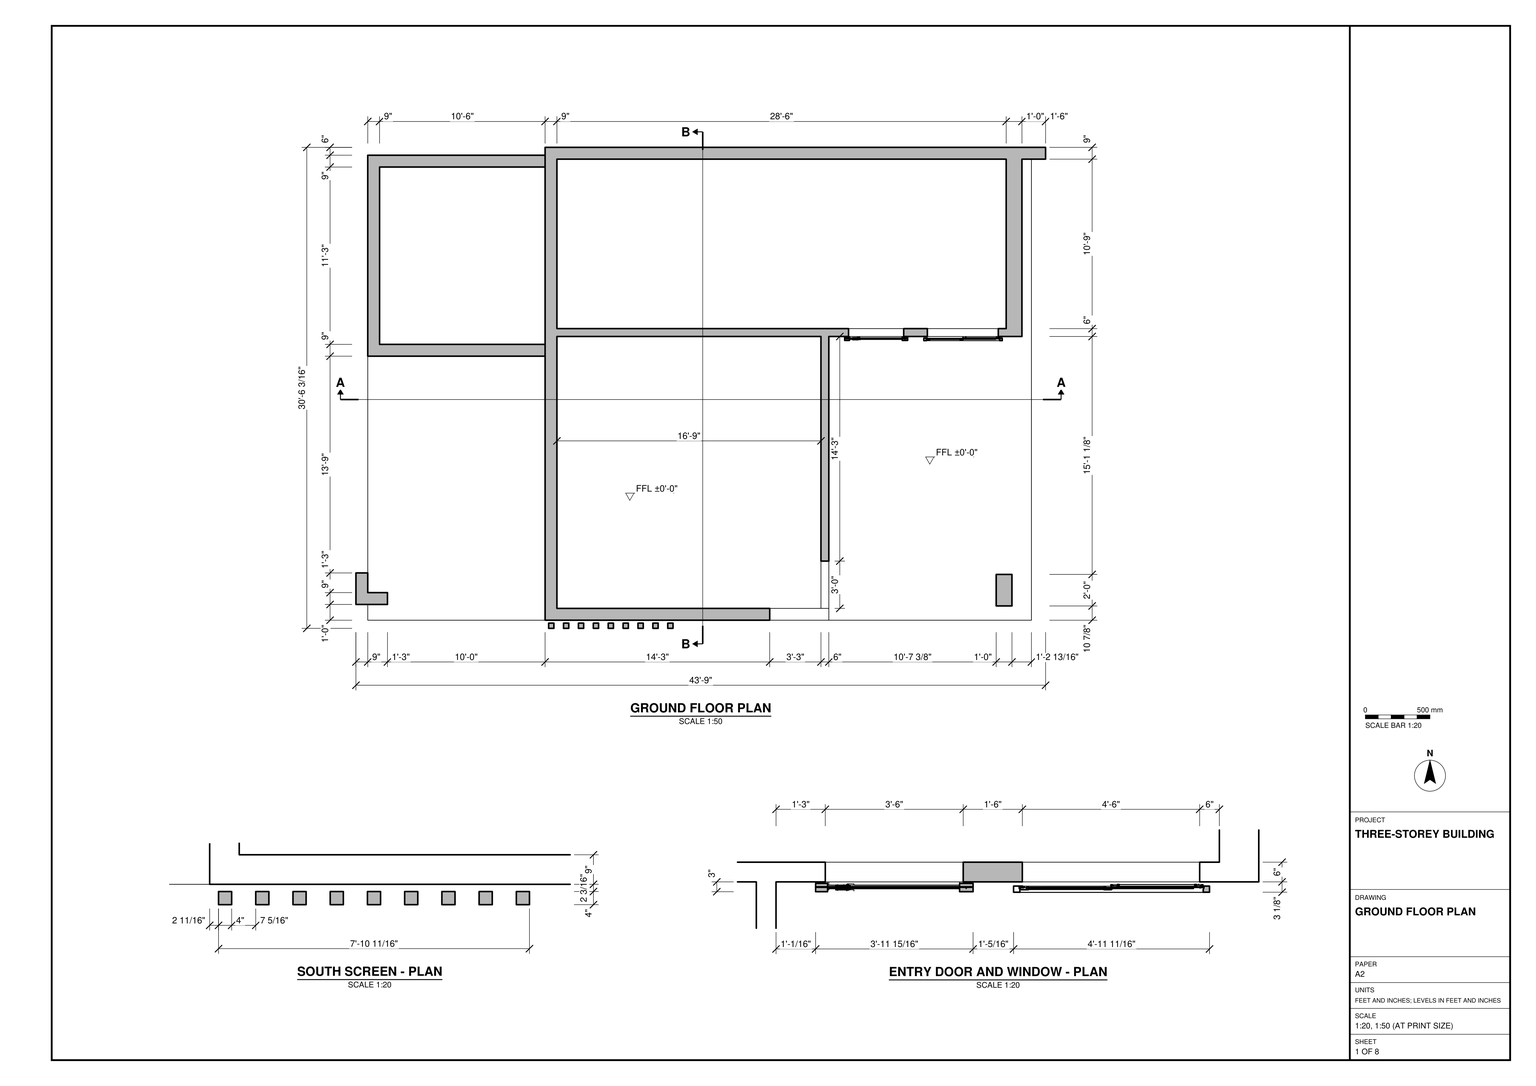
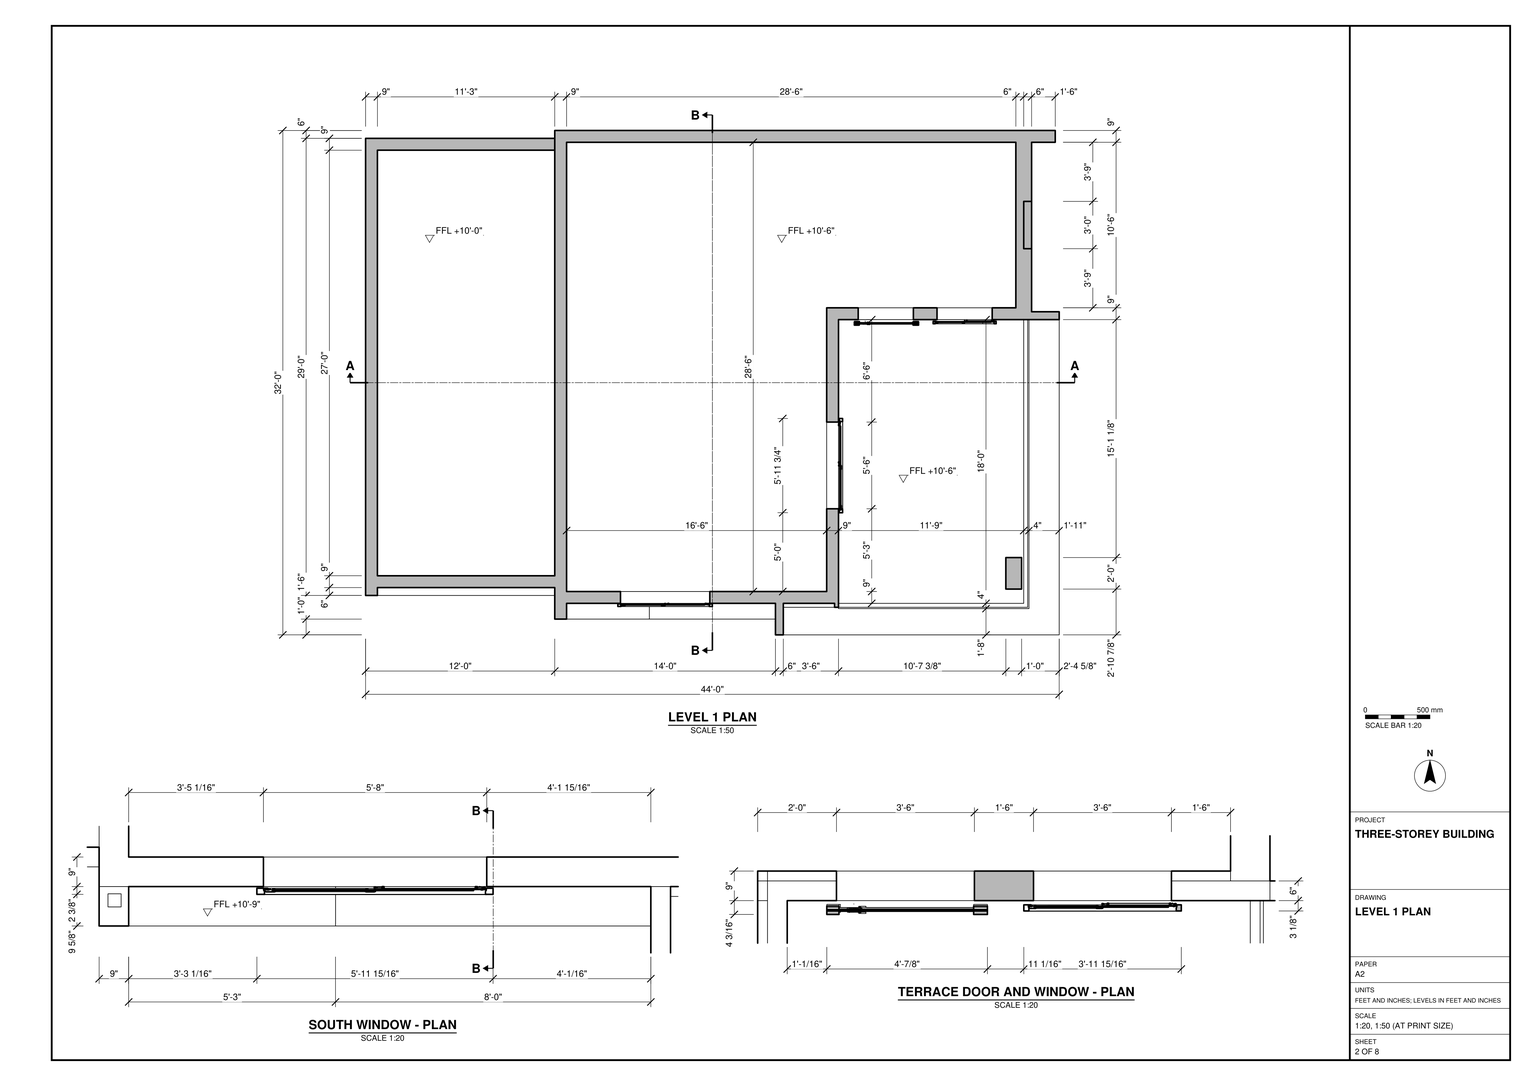
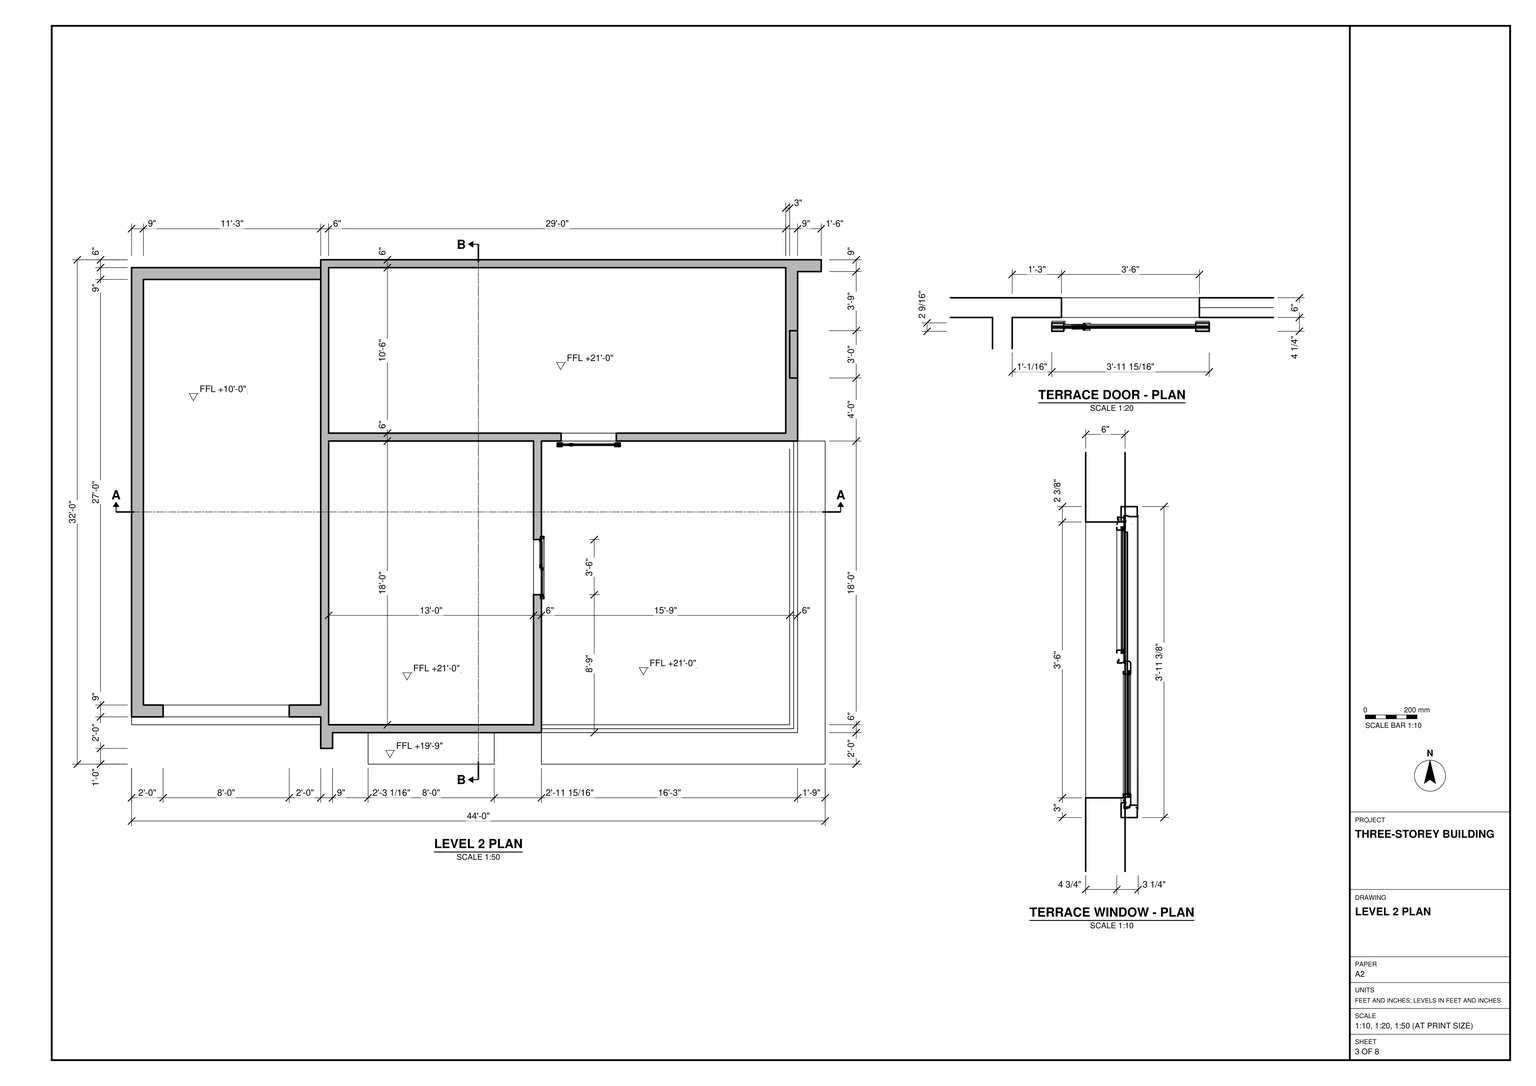
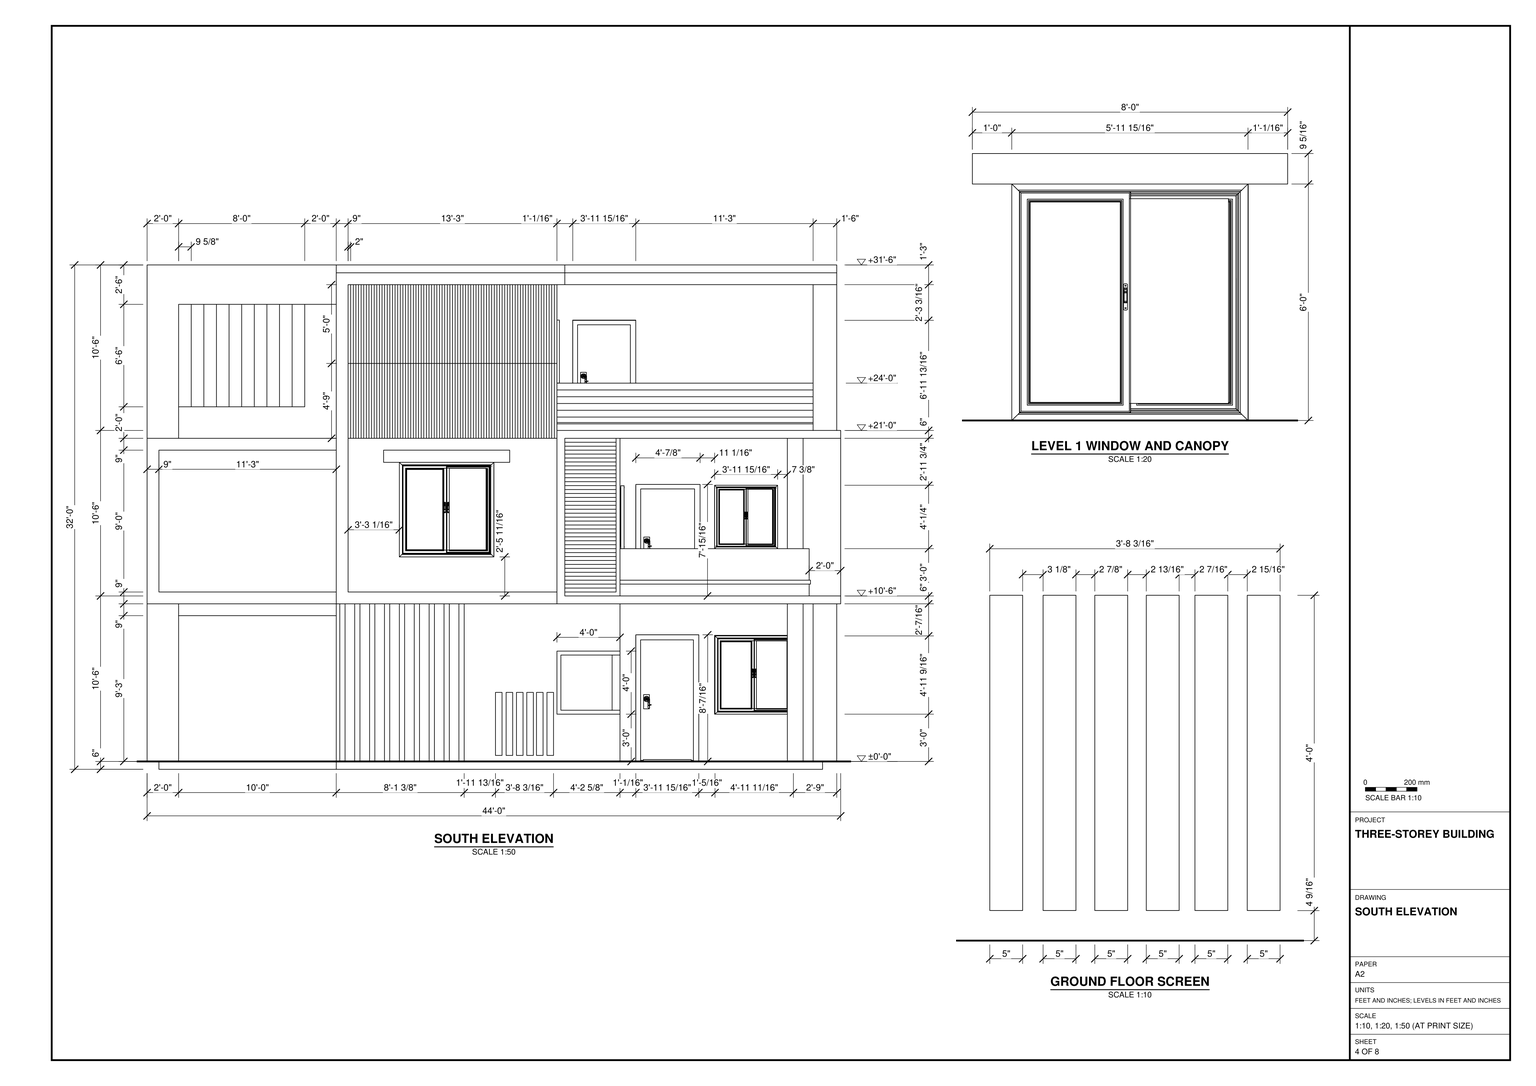
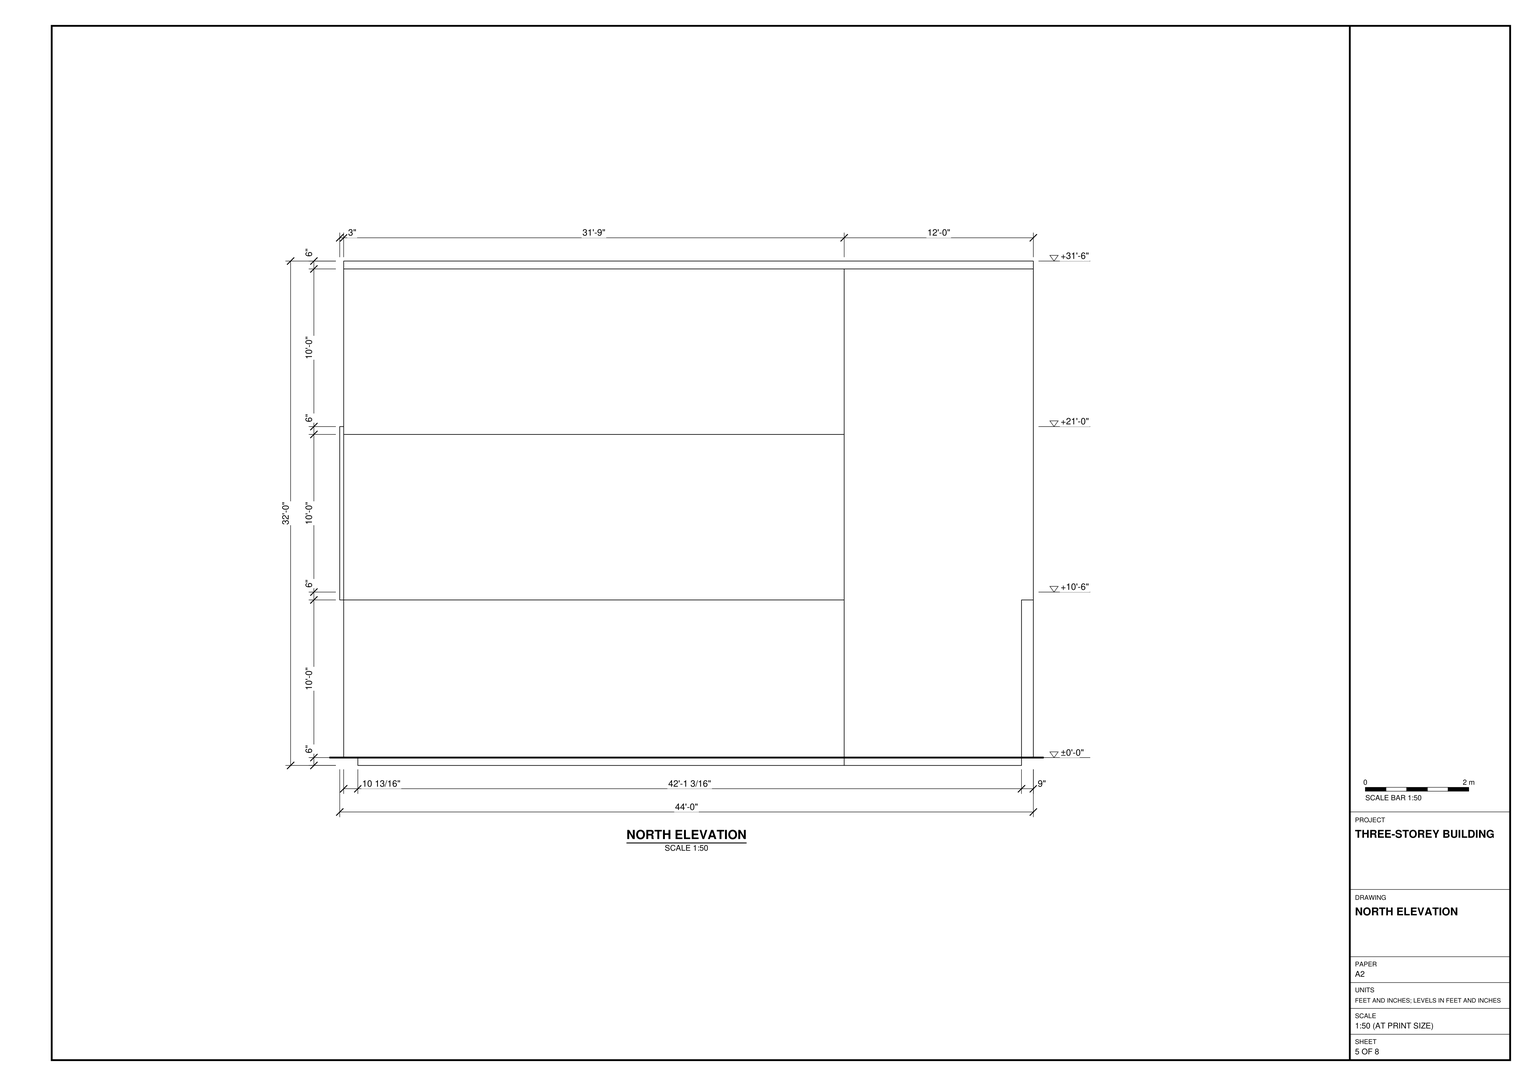
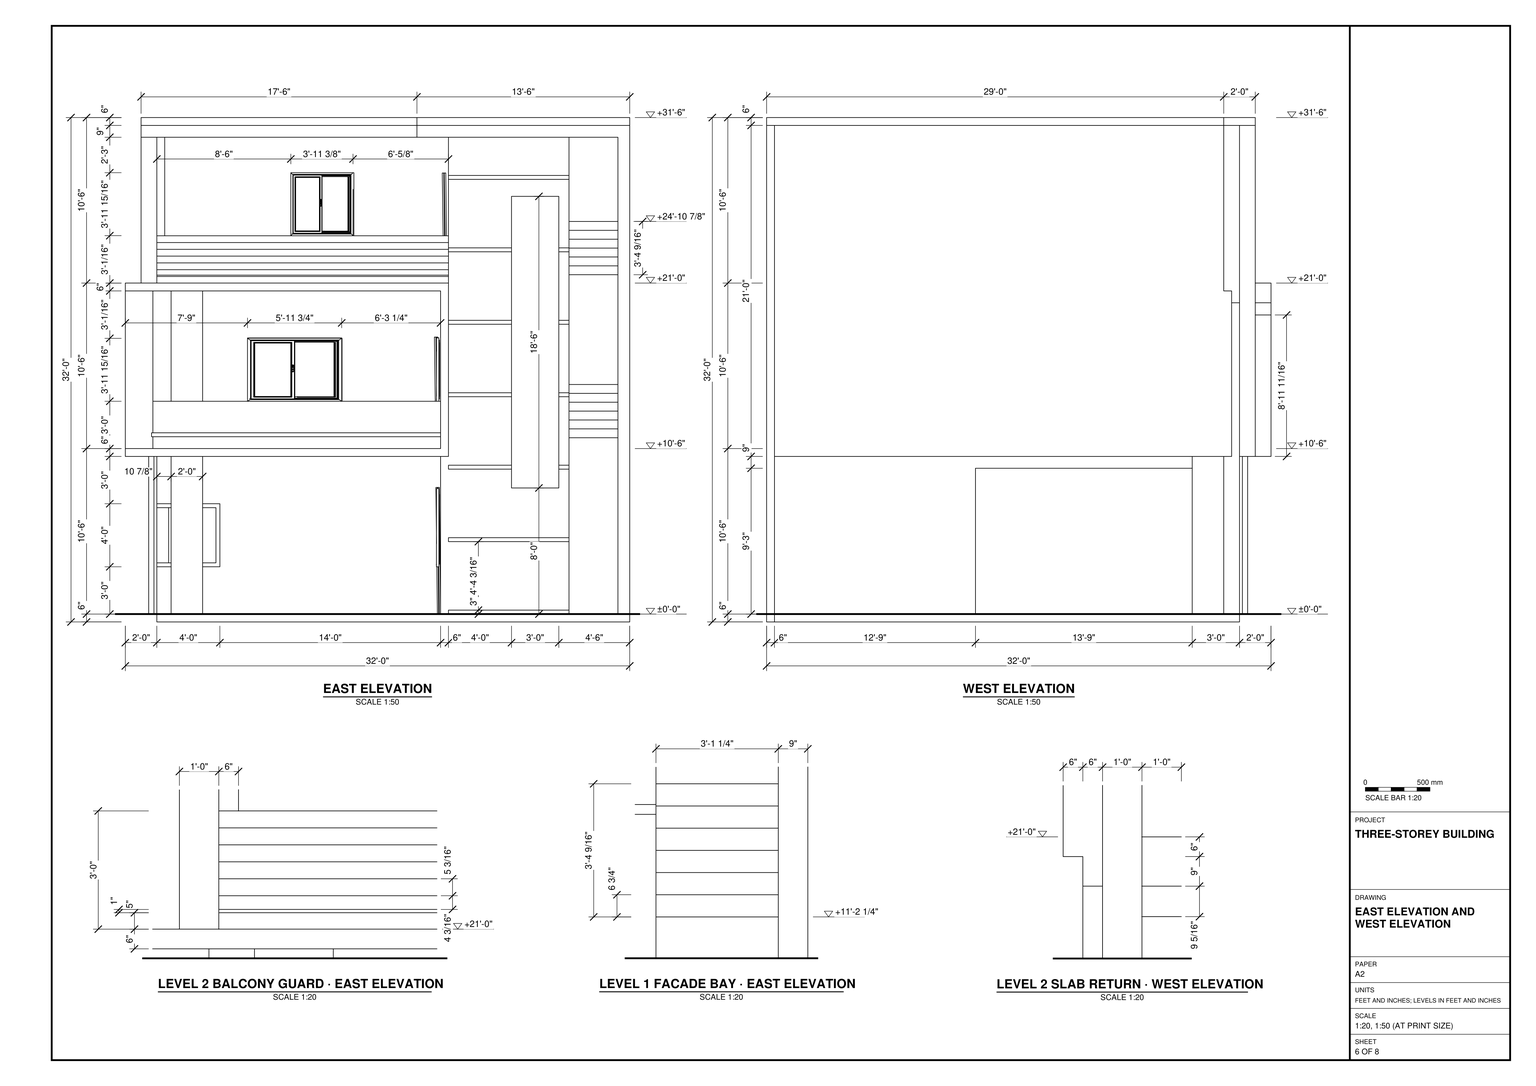
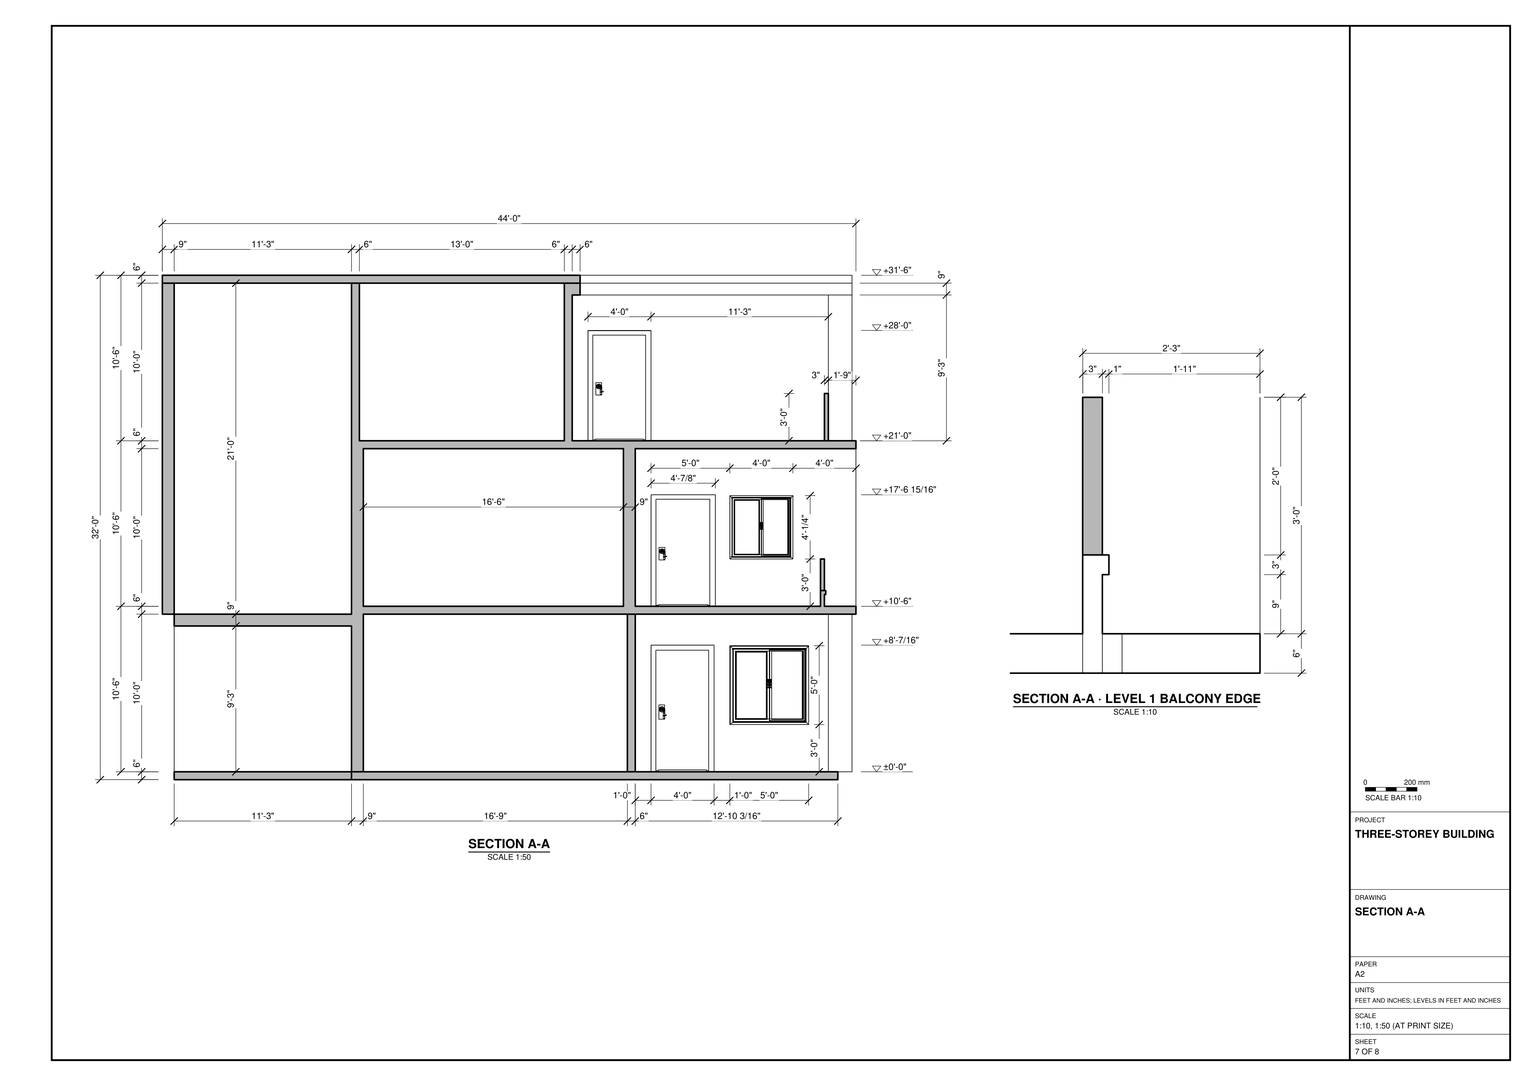
Build the three-storey building in SketchUp from task_files/diagram_01.pdf. Work in feet and inches. The overall dimensions are 44'-0" east to west, 32'-0" north to south and 32'-0" high. Set the main finished floor levels at ±0'-0", +10'-6" and +21'-0". Keep the lower western bay at the separate +10'-0" level shown on the upper plans.

Start with the long north room, the central room extending south, and the smaller northwest enclosure. Follow the wall thicknesses on each plan, including the 9" walls of the northwest enclosure and the 6" walls around the upper south room. Model the freestanding ground-floor supports and the row of spaced screen members outside the south wall. Set the entry door and adjacent window into the wall facing the open southeast bay.

Model the floor slabs, terrace edges and roof to the outlines on the sheets. The central room narrows on the top storey, leaving a wider southeast terrace. Use the enlarged details to locate the framed doors and windows in the terrace walls and the window in the south wall below.

Keep walls, slabs and roof elements as separate groups or components. Keep any furniture or joinery pieces separate and use components for repeated parts such as the screen members. Any decor or loose items shown may be suitable library components. Save one SketchUp model as output_files/building_with_stepped_terraces_and_south_screen.skp.

# SketchUp Ruby script. Lengths in inches.
U = 1.inch
M = Sketchup.active_model
def pt(a) = Geom::Point3d.new(a.map { |v| v * U })
def face(e, loops, mat)
  f = e.add_face(loops[0].map { |a| pt(a) })
  loops[1..].each { |l| e.add_face(l.map { |a| pt(a) }).erase! }
  f.material = f.back_material = mat if mat
  f
end
# faces: each face lists its corners as indices into pts; further lists are holes
def faces(e, pts, list, mat = nil) = list.each { |f| face(e, (f[0].is_a?(Array) ? f : [f]).map { |l| l.map { |i| pts[i] } }, mat) }
# xy, xz, yz: faces in a plane at the given z, y or x. An outline is a flat list of corners, or four numbers for a rectangle; further outlines are holes
def ring(l) = l.size == 4 ? [[l[0], l[1]], [l[2], l[1]], [l[2], l[3]], [l[0], l[3]]] : l.each_slice(2).to_a
def flat(e, list, mat, &to3) = list.each { |f| face(e, (f[0].is_a?(Array) ? f : [f]).map { |l| ring(l).map { |u, v| to3.(u, v) } }, mat) }
def xy(e, z, list, mat = nil) = flat(e, list, mat) { |x, y| [x, y, z] }
def xz(e, y, list, mat = nil) = flat(e, list, mat) { |x, z| [x, y, z] }
def yz(e, x, list, mat = nil) = flat(e, list, mat) { |y, z| [x, y, z] }
def lines(e, pts, list) = list.each { |a, b| e.add_line(pt(pts[a]), pt(pts[b])) }
# prism: a flat outline (further loops are holes) pulled along v
def prism(e, loops, v, mat = nil)
  f = face(e, loops, mat); d = Geom::Vector3d.new(v.map { |x| x * U })
  f.pushpull(f.normal.samedirection?(d) ? d.length : -d.length)
end
def box(e, o, s, mat = nil) = prism(e, [[o, [o[0] + s[0], o[1], o[2]], [o[0] + s[0], o[1] + s[1], o[2]], [o[0], o[1] + s[1], o[2]]]], [0, 0, s[2]], mat)
def at(x, y, z, deg = 0) = Geom::Transformation.translation(pt([x, y, z])) * Geom::Transformation.rotation(ORIGIN, Z_AXIS, deg.degrees)
def axes(o, x, y, z) = Geom::Transformation.new([*x, 0, *y, 0, *z, 0, *pt(o).to_a, 1])
def part(name) = M.definitions.add(name)
# library, detail: a bought-in or finely detailed component or shape, given as its bounding box
def library(name, o, s) = part(name).tap { |d| box(d.entities, o, s) }
def detail(e, o, s) = box(e.add_group.entities, o, s)
def put(e, d, t, mat = nil) = e.add_instance(d, t).tap { |i| i.material = mat if mat }
def group(e, t, mat = nil) = e.add_group.tap { |g| g.transformation = t; g.material = mat if mat }.entities
root = M.entities
M.materials.add("C03_Honey_Glow").color = [255, 178, 101]
M.materials.add("C05_Golden_Blaze").color = [255, 123, 0]
M.materials.add("C08_Toffee_Ember").color = [102, 51, 0]
M.materials.add("Carpet_04_1K").color = [43, 65, 85]
M.materials.add("D08_Bronzed_Mustard").color = [102, 74, 0]
M.materials.add("Denim_03_1K").color = [93, 106, 119]
M.materials.add("E01_Mint_Frost").color = [255, 255, 204]
M.materials.add("Glass_Basic_01").color = [186, 162, 180]
M.materials["Glass_Basic_01"].alpha = 0.25
M.materials.add("Gravel_01_1K").color = [153, 136, 116]
M.materials.add("M06_Steel_Smoke").color = [86, 86, 86]
M.materials.add("Plywood_01_1K").color = [125, 96, 64]
M.materials.add("ThomThom - Buttons2").color = [40, 40, 43]
M.materials.add("[Color_000]").color = [255, 255, 255]
c1 = library("porta+4",[0.2,-5.42,1.33],[46.55,4.72,83.21])
c2 = library("mesh-165",[-1596.32,-2661.67,-39.91],[1702.88,1739.15,82.5])
c3 = part("Group15")
put(c3.entities,c2,at(294.66,859.51,3.5))
xy(root,-6,[[144,24,514.22,384]])
xy(root,0,[[[144,24,360,24,360,240,507,240,507,384,144,384],[153,246,495,375],[153,33,354,240]],[360,24,514.22,24,514.22,384,507,384,507,240,360,240],[153,33,354,240],[153,246,495,375]])
xz(root,24,[[144,-6,514.22,0]])
xz(root,384,[[144,-6,514.22,0]])
yz(root,144,[[24,-6,384,0]])
yz(root,514.22,[[24,-6,384,0]])
p = [[144,384,372],[144,246,372],[504,246,372],[504,384,372],[144,246,378],[153,18,246],
  [153,18,237]]
lines(root,p,[[0,1],[1,2],[2,3],[3,0],[1,4],[5,6]])
g1 = group(root,at(144,24,0))
xy(g1,-6,[[-135,0,0,354]])
xy(g1,0,[[14.03,-6.2,18.03,-2.2],[25.37,-6.2,29.37,-2.2],[36.7,-6.2,40.7,-2.2],[48.04,-6.2,52.04,-2.2],[59.375,-6.2,63.375,-2.2],
  [70.71,-6.2,74.71,-2.2],[82.05,-6.2,86.05,-2.2],[93.38,-6.2,97.38,-2.2],[-135,0,0,0,0,201,-135,201,-135,21,-120,21,-120,12,-135,12],[[0,0,0,360,381,360,381,351,363,351,363,216,216,216,216,0],[9,222,351,351],[9,9,210,216]],
  [343.39,10.86,355.39,34.86],[-144,12,-135,36],[-135,12,-120,21],[-135,201,-135,354,0,354,0,345,-126,345,-126,210,0,210,0,201],[-126,210,0,345]])
xy(g1,0.4,[[2.7,-6.2,6.7,-2.2]])
xy(g1,3,[[231,216,273,222]])
xy(g1,39,[[171,0,216,9],[210,9,216,45],[291,216,345,222]])
xy(g1,81,[[171,0,216,9],[210,9,216,45]])
xy(g1,93,[[231,216,273,222],[291,216,345,222]])
xy(g1,95.99,[[357,270,363,306]])
xy(g1,111,[[-135,21,-126,201],[-126,210,0,345]],"E01_Mint_Frost")
xy(g1,111,[[-126,21,0,201]],"[Color_000]")
xy(g1,120,[[[0,-12,168,0],[2.7,-6.2,6.7,-2.2],[14.03,-6.2,18.03,-2.2],[25.37,-6.2,29.37,-2.2],[36.7,-6.2,40.7,-2.2],[48.04,-6.2,52.04,-2.2],[59.375,-6.2,63.375,-2.2],[70.71,-6.2,74.71,-2.2],[82.05,-6.2,86.05,-2.2],[93.38,-6.2,97.38,-2.2]],[-144,6,-144,12,-120,12,-120,21,0,21,0,6],[9,9,210,216],[210,9,216,9,216,216,363,216,363,222,210,222],[-144,36,-135,354],
  [9,216,210,222],[9,222,210,351],[210,222,351,351],[9,351,210,360]])
xy(g1,120,[[241.125,19.91,249.125,139.91],[263.3,19.91,271.3,139.91],[285.48,19.91,293.48,139.91],[307.66,19.91,315.66,139.91],[329.83,19.91,337.83,139.91]],"C03_Honey_Glow")
xy(g1,120,[[[168,-24,168,0,216,0,216,216,363,216,363,222,384,222,384,-24],[241.125,19.91,249.125,139.91],[263.3,19.91,271.3,139.91],[285.48,19.91,293.48,139.91],[307.66,19.91,315.66,139.91],[329.83,19.91,337.83,139.91]]],"Carpet_04_1K")
xy(g1,120,[[-135,21,0,345]],"E01_Mint_Frost")
xy(g1,126,[[174,-24,384,-24,384,216,360,216,360,-3,174,-3],[216,0,357,216],[9,9,207,9,207,225,351,225,351,351,9,351]])
xy(g1,129,[[9,-12,72,0],[72,-12,168,0],[-135,6,0,12],[231,216,273,225]])
xy(g1,129,[[174,-3,213,0]],"C08_Toffee_Ember")
xy(g1,132,[[174,-3,213,0]],"C08_Toffee_Ember")
xy(g1,135,[[216,-4,216,-3,360,-3,360,216,361,216,361,-4]])
xy(g1,135,[[174,-3,213,0]],"C08_Toffee_Ember")
xy(g1,138,[[216,-4,361,-4,361,216,360,216,360,-3,216,-3],[216,-3,360,-3,360,216,357,216,357,0,216,0]])
xy(g1,138,[[174,-3,213,0]],"C08_Toffee_Ember")
xy(g1,141,[[174,-3,213,0]],"C08_Toffee_Ember")
xy(g1,144,[[174,-3,213,0]],"C08_Toffee_Ember")
xy(g1,147,[[174,-3,213,0]],"C08_Toffee_Ember")
xy(g1,150,[[174,-3,213,0]],"C08_Toffee_Ember")
xy(g1,153,[[174,-3,213,0]],"C08_Toffee_Ember")
xy(g1,156,[[174,-3,213,0]],"C08_Toffee_Ember")
xy(g1,157.71,[[50.04,0,118.04,9]])
xy(g1,159,[[174,-3,213,0]],"C08_Toffee_Ember")
xy(g1,162,[[216,-3,360,-3,360,216,357,216,357,0,216,0]])
xy(g1,162,[[174,-3,213,0]],"C08_Toffee_Ember")
xy(g1,165,[[207,72,216,138],[291,216,333,225]])
xy(g1,165,[[174,-3,213,0]],"C08_Toffee_Ember")
xy(g1,168,[[174,-3,213,0]],"C08_Toffee_Ember")
xy(g1,171,[[174,-3,213,0]],"C08_Toffee_Ember")
xy(g1,174,[[174,-3,213,0]],"C08_Toffee_Ember")
xy(g1,177,[[174,-3,213,0]],"C08_Toffee_Ember")
xy(g1,180,[[174,-3,213,0]],"C08_Toffee_Ember")
xy(g1,183,[[174,-3,213,0]],"C08_Toffee_Ember")
xy(g1,186,[[174,-3,213,0]],"C08_Toffee_Ember")
xy(g1,189,[[174,-3,213,0]],"C08_Toffee_Ember")
xy(g1,192,[[174,-3,213,0]],"C08_Toffee_Ember")
xy(g1,195,[[174,-3,213,0]],"C08_Toffee_Ember")
xy(g1,198,[[174,-3,213,0]],"C08_Toffee_Ember")
xy(g1,201,[[174,-3,213,0]],"C08_Toffee_Ember")
xy(g1,204,[[174,-3,213,0]],"C08_Toffee_Ember")
xy(g1,207,[[207,72,216,138],[231,216,273,225],[291,216,333,225]])
xy(g1,207,[[174,-3,213,0]],"C08_Toffee_Ember")
xy(g1,210,[[174,-3,213,0]],"C08_Toffee_Ember")
xy(g1,213,[[174,-3,213,0]],"C08_Toffee_Ember")
xy(g1,216,[[174,-3,213,0]],"C08_Toffee_Ember")
xy(g1,219,[[174,-3,213,0]],"C08_Toffee_Ember")
xy(g1,222,[[174,-3,213,0]],"C08_Toffee_Ember")
xy(g1,225,[[174,-3,213,0]],"C08_Toffee_Ember")
xy(g1,225.71,[[50.04,0,118.04,9]])
xy(g1,227.71,[[36.04,-24,132.04,0]],"E01_Mint_Frost")
xy(g1,228,[[174,-3,213,0]],"C08_Toffee_Ember")
xy(g1,231,[[174,-3,213,0]],"C08_Toffee_Ember")
xy(g1,234,[[174,-3,213,0]],"C08_Toffee_Ember")
xy(g1,237,[[36.04,-24,132.04,0],[-135,6,0,12]])
xy(g1,237,[[174,-3,213,0]],"C08_Toffee_Ember")
xy(g1,240,[[174,-3,213,0]],"C08_Toffee_Ember")
xy(g1,243,[[174,-3,213,0]],"C08_Toffee_Ember")
xy(g1,246,[[213,-3,216,-3,216,9,9,9,9,0,213,0],[-144,6,0,12],[9,9,9,351,351,351,351,225,207,225,207,9]])
xy(g1,246,[[241.125,19.91,249.125,139.91],[263.3,19.91,271.3,139.91],[285.48,19.91,293.48,139.91],[307.66,19.91,315.66,139.91],[329.83,19.91,337.83,139.91]],"C03_Honey_Glow")
xy(g1,246,[[[174,-24,174,0,213,0,213,-3,216,-3,216,216,384,216,384,-24],[241.125,19.91,249.125,139.91],[263.3,19.91,271.3,139.91],[285.48,19.91,293.48,139.91],[307.66,19.91,315.66,139.91],[329.83,19.91,337.83,139.91],[343.39,10.86,355.39,34.86]]],"Carpet_04_1K")
xy(g1,252,[[168,-24,384,-24,384,222,363,222,363,0,168,0],[168,0,363,0,363,3,360,3,168,2.98],[168,2.98,360,3,168,3],[168,3,360,222],[360,3,363,222],
  [6,6,162,222],[6,228,354,354]])
xy(g1,255,[[183,222,225,228]])
xy(g1,270,[[-120,12,-24,21]])
xy(g1,288,[[168,0,363,0,363,222,360,222,360,3,168,2.98]])
xy(g1,291,[[162,105,168,147]],"C08_Toffee_Ember")
xy(g1,318,[[357,270,363,306]])
xy(g1,333,[[183,222,225,228]])
xy(g1,333,[[162,105,168,147]],"C08_Toffee_Ember")
xy(g1,348,[[-120,12,-24,21]])
xy(g1,363,[[9,-12,174,0],[168,0,174,6],[168,6,174,216],[174,198,174,222,363,222,363,351,381,351,381,198],[168,216,174,222]])
xy(g1,372,[[6,-12,162,6],[162,-12,174,21],[6,6,162,21],[-144,21,-135,354],[-135,21,0,345],
  [0,21,6,222],[6,21,162,216],[162,21,174,216],[174,198,381,198,381,228,6,228,6,345,0,345,0,222,174,222],[6,216,162,222],
  [162,216,174,222],[6,228,354,345],[354,228,381,345],[-135,345,0,354],[0,345,6,360],
  [6,345,354,354],[354,345,381,360],[-144,354,-135,360],[-135,354,0,360],[6,354,174,360],
  [174,354,354,360]])
xy(g1,378,[[0,-12,174,-12,174,198,381,198,381,360,-144,360,-144,12,0,12]])
xz(g1,-24,[[168,120,384,120,384,126,174,126,174,246,384,246,384,252,168,252]])
xz(g1,-24,[[36.04,227.71,132.04,237]],"[Color_000]")
xz(g1,-12,[[0,120,168,120,168,129,9,129,9,363,174,363,174,372,0,372],[0,372,174,378]])
xz(g1,-6.2,[[14.03,0,18.03,120],[25.37,0,29.37,120],[36.7,0,40.7,120],[48.04,0,52.04,120],[59.375,0,63.375,120],
  [70.71,0,74.71,120],[82.05,0,86.05,120],[93.38,0,97.38,120],[2.7,0.4,6.7,120]],"M06_Steel_Smoke")
xz(g1,-4,[[216,135,361,138]])
xz(g1,-3,[[174,126,216,126,216,246,213,246,213,129,174,129],[174,132,213,135],[174,138,213,141],[174,144,213,147],[174,150,213,153],
  [174,156,213,159],[174,162,213,165],[174,168,213,171],[174,174,213,177],[174,180,213,183],
  [174,186,213,189],[174,192,213,195],[174,198,213,201],[174,204,213,207],[174,210,213,213],
  [174,216,213,219],[174,222,213,225],[174,228,213,231],[174,234,213,237],[174,240,213,243]],"C08_Toffee_Ember")
xz(g1,-3,[[216,126,360,135]],"Denim_03_1K")
xz(g1,-3,[[216,138,360,162]],"Glass_Basic_01")
xz(g1,-2.2,[[14.03,0,18.03,120],[25.37,0,29.37,120],[36.7,0,40.7,120],[48.04,0,52.04,120],[59.375,0,63.375,120],
  [70.71,0,74.71,120],[82.05,0,86.05,120],[93.38,0,97.38,120],[2.7,0.4,6.7,120]])
xz(g1,0,[[-135,-6,0,0],[216,126,357,138],[213,147,216,150],[[48.04,155.71,120.04,227.71],[50.04,157.71,118.04,225.71]]])
xz(g1,0,[[[0,0,216,0,216,36,168,36,168,84,216,84,216,120,0,120],[121.2,4.58,126.2,52.58],[129.32,4.58,134.32,52.58],[137.19,4.58,142.19,52.58],[145.03,4.58,150.03,52.58],[152.4375,4.58,157.4375,52.58],[160.4,4.58,165.4,52.58]]],"C03_Honey_Glow")
xz(g1,0,[[174,129,213,132],[174,135,213,138],[174,141,213,144],[174,147,213,150],[174,153,213,156],
  [174,159,213,162],[174,165,213,168],[174,171,213,174],[174,177,213,180],[174,183,213,186],
  [174,189,213,192],[174,195,213,198],[174,201,213,204],[174,207,213,210],[174,213,213,216],
  [174,219,213,222],[174,225,213,228],[174,231,213,234],[174,237,213,240],[174,243,213,246],
  [9,246,10.99,303],[10.99,246,12.97,303],[12.97,246,14.96,303],[14.96,246,16.95,303],[16.95,246,18.9375,303],
  [18.9375,246,20.92,303],[20.92,246,22.91,303],[22.91,246,24.9,303],[24.9,246,26.89,303],[26.89,246,28.875,303],
  [28.875,246,30.86,303],[30.86,246,32.85,303],[32.85,246,34.84,303],[34.84,246,36.83,303],[36.83,246,38.8125,303],
  [38.8125,246,40.8,303],[40.8,246,42.79,303],[42.79,246,44.78,303],[44.78,246,46.76,303],[46.76,246,48.75,303],
  [48.75,246,50.74,303],[50.74,246,52.72,246,52.73,303,50.74,303],[52.72,246,54.71,246,54.71,303,52.73,303],[54.71,246,56.7,303],[56.7,246,58.6875,303],
  [58.6875,246,60.67,246,60.68,303,58.6875,303],[60.67,246,62.66,246,62.66,303,60.68,303],[62.66,246,64.65,303],[64.65,246,66.64,303],[66.64,246,68.625,303],
  [68.625,246,70.61,303],[70.61,246,72.6,303],[72.6,246,74.59,303],[74.59,246,76.58,303],[76.58,246,78.5625,303],
  [78.5625,246,80.55,303],[80.55,246,82.54,303],[82.54,246,84.52,246,84.53,303,82.54,303],[84.52,246,86.51,246,86.51,303,84.53,303],[86.51,246,88.5,303],
  [88.5,246,90.49,303],[90.49,246,92.47,246,92.48,303,90.49,303],[92.47,246,94.46,246,94.46,303,92.48,303],[94.46,246,96.45,303],[96.45,246,98.4375,303],
  [98.4375,246,100.42,303],[100.42,246,102.41,303],[102.41,246,104.4,303],[104.4,246,106.39,303],[106.39,246,108.375,303],
  [108.375,246,110.36,303],[110.36,246,112.35,303],[112.35,246,114.34,303],[114.34,246,116.32,246,116.33,303,114.34,303],[116.32,246,118.3125,246,118.3125,303,116.33,303],
  [118.3125,246,120.3,303],[120.3,246,122.29,303],[122.29,246,124.27,246,124.28,303,122.29,303],[124.27,246,126.26,246,126.26,303,124.28,303],[126.26,246,128.25,303],
  [128.25,246,130.24,303],[130.24,246,132.22,303],[132.22,246,134.21,303],[134.21,246,136.2,303],[136.2,246,138.1875,303],
  [138.1875,246,140.17,303],[140.17,246,142.16,303],[142.16,246,144.15,303],[144.15,246,146.14,303],[146.14,246,148.125,303],
  [148.125,246,150.11,303],[150.11,246,152.1,303],[152.1,246,154.09,303],[154.09,246,156.08,303],[156.08,246,158.0625,303],
  [158.0625,246,160.05,303],[160.05,246,162.04,303],[162.04,246,164.03,303],[164.03,246,166.01,303],[166.01,246,168,303],
  [9,303,10.99,363],[10.99,303,12.97,363],[12.97,303,14.96,363],[14.96,303,16.95,363],[16.95,303,18.9375,363],
  [18.9375,303,20.92,363],[20.92,303,22.91,363],[22.91,303,24.9,363],[24.9,303,26.89,363],[26.89,303,28.875,363],
  [28.875,303,30.86,363],[30.86,303,32.85,363],[32.85,303,34.84,363],[34.84,303,36.83,363],[36.83,303,38.8125,363],
  [38.8125,303,40.8,363],[40.8,303,42.79,363],[42.79,303,44.78,363],[44.78,303,46.76,363],[46.76,303,48.75,363],
  [48.75,303,50.74,363],[50.74,303,52.73,363],[52.73,303,54.71,363],[54.71,303,56.7,363],[56.7,303,58.6875,363],
  [58.6875,303,60.68,363],[60.68,303,62.66,363],[62.66,303,64.65,363],[64.65,303,66.64,363],[66.64,303,68.625,363],
  [68.625,303,70.61,363],[70.61,303,72.6,363],[72.6,303,74.59,363],[74.59,303,76.58,363],[76.58,303,78.5625,363],
  [78.5625,303,80.55,363],[80.55,303,82.54,363],[82.54,303,84.53,363],[84.53,303,86.51,363],[86.51,303,88.5,363],
  [88.5,303,90.49,363],[90.49,303,92.48,363],[92.48,303,94.46,363],[94.46,303,96.45,363],[96.45,303,98.4375,363],
  [98.4375,303,100.42,363],[100.42,303,102.41,363],[102.41,303,104.4,363],[104.4,303,106.39,363],[106.39,303,108.375,363],
  [108.375,303,110.36,363],[110.36,303,112.35,363],[112.35,303,114.34,363],[114.34,303,116.33,363],[116.33,303,118.3125,363],
  [118.3125,303,120.3,363],[120.3,303,122.29,363],[122.29,303,124.28,363],[124.28,303,126.26,363],[126.26,303,128.25,363],
  [128.25,303,130.24,363],[130.24,303,132.22,363],[132.22,303,134.21,363],[134.21,303,136.2,363],[136.2,303,138.1875,363],
  [138.1875,303,140.17,363],[140.17,303,142.16,363],[142.16,303,144.15,363],[144.15,303,146.14,363],[146.14,303,148.125,363],
  [148.125,303,150.11,363],[150.11,303,152.1,363],[152.1,303,154.09,363],[154.09,303,156.08,363],[156.08,303,158.0625,363],
  [158.0625,303,160.05,363],[160.05,303,162.04,363],[162.04,303,164.03,363],[164.03,303,166.01,363],[166.01,303,168,363]],"C08_Toffee_Ember")
xz(g1,0,[[168,36,216,36,216,39,171,39,171,81,216,81,216,84,168,84]],"D08_Bronzed_Mustard")
xz(g1,0,[[216,138,357,162],[168,252,363,257],[168,258,363,262.17],[168,262.17,363,267.33],[168,267.33,363,272.5],
  [168,272.5,363,277.67],[168,277.67,363,282.83],[168,282.83,363,288]],"Glass_Basic_01")
xz(g1,0,[[121.2,4.58,126.2,52.58],[129.32,4.58,134.32,52.58],[137.19,4.58,142.19,52.58],[145.03,4.58,150.03,52.58],[152.4375,4.58,157.4375,52.58],
  [160.4,4.58,165.4,52.58]],"M06_Steel_Smoke")
xz(g1,0,[[168,257,363,258]],"ThomThom - Buttons2")
xz(g1,0,[[[9,129,168,246],[48.04,155.71,48.04,227.71,36.04,227.71,36.04,237,132.04,237,132.04,227.71,120.04,227.71,120.04,155.71]]],"[Color_000]")
xz(g1,6,[[-144,120,0,120,0,129,-135,129,-135,237,0,237,0,246,-144,246],[6,252,162,372]])
xz(g1,9,[[9,0,9,120,210,120,210,81,171,81,171,39,210,39,210,0],[[9,126,207,246],[50.04,157.71,118.04,225.71]]])
xz(g1,10.86,[[343.39,0,355.39,246]])
xz(g1,12,[[-144,0,-120,120],[-144,246,-120,246,-120,348,0,348,0,378,-144,378]],"Gravel_01_1K")
xz(g1,12,[[-135,129,0,237]],"Plywood_01_1K")
xz(g1,12,[[-120,246,0,246,0,348,-24,348,-24,270,-120,270]],"[Color_000]")
xz(g1,21,[[-135,0,-120,111],[-135,111,-120,120],[[-135,120,0,372],[-120,270,-24,348]]])
xz(g1,21,[[-120,111,0,120]],"[Color_000]")
xz(g1,34.86,[[343.39,0,355.39,246]])
xz(g1,36,[[-144,0,-135,120]])
xz(g1,45,[[210,39,216,81]])
xz(g1,72,[[207,165,216,207]])
xz(g1,105,[[162,291,168,333]],"C08_Toffee_Ember")
xz(g1,138,[[207,165,216,207]])
xz(g1,147,[[162,291,168,333]],"C08_Toffee_Ember")
xz(g1,198,[[174,363,381,372],[174,372,381,378]])
xz(g1,201,[[-135,0,0,111]],"[Color_000]")
xz(g1,210,[[-126,0,0,111]],"E01_Mint_Frost")
xz(g1,216,[[[228,0,276,96],[231,3,273,93]],[[288,36,348,96],[291,39,345,93]],[[228,126,276,210],[231,129,273,207]],[357,138,360,162],[[288,162,336,210],[291,165,333,207]]])
xz(g1,216,[[9,0,210,120]],"C05_Golden_Blaze")
xz(g1,216,[[[216,0,228,0,228,96,276,96,276,0,363,0,363,120,216,120],[288,36,348,96]]],"Denim_03_1K")
xz(g1,216,[[[216,126,228,126,228,210,276,210,276,126,357,126,357,162,360,162,360,138,361,138,361,135,360,135,360,126,384,126,384,246,216,246],[288,162,336,210]]],"[Color_000]")
xz(g1,222,[[9,0,216,120],[[216,0,351,120],[231,3,273,93],[291,39,345,93]],[363,120,384,252],[6,252,162,372],[[180,252,228,336],[183,255,225,333]],
  [360,252,363,288]])
xz(g1,222,[[168,252,180,252,180,336,228,336,228,252,360,252,360,288,363,288,363,363,168,363]],"[Color_000]")
xz(g1,225,[[[207,126,351,246],[231,129,273,207],[291,165,333,207]]])
xz(g1,228,[[[6,252,354,372],[183,255,225,333]]])
xz(g1,270,[[357,95.99,363,318]])
xz(g1,306,[[357,95.99,363,318]])
xz(g1,345,[[-126,0,0,111]],"E01_Mint_Frost")
xz(g1,345,[[-135,120,0,372]],"[Color_000]")
xz(g1,351,[[363,0,381,363],[9,126,351,246]])
xz(g1,351,[[9,0,351,120]],"C05_Golden_Blaze")
xz(g1,354,[[-135,-6,0,0],[-135,0,-135,120,-144,120,-144,372,0,372,0,0],[6,252,354,372]])
xz(g1,360,[[0,0,381,120],[0,120,381,246],[0,246,381,372],[-144,372,381,378]])
yz(g1,-144,[[12,0,36,120],[12,372,360,378]])
yz(g1,-144,[[6,120,6,246,12,246,12,372,354,372,354,120]],"[Color_000]")
yz(g1,-135,[[0,-6,354,0],[21,0,36,111],[201,0,201,111,36,111,36,120,354,120,354,0],[21,111,36,120],[21,120,345,372],
  [6,129,12,237]])
yz(g1,-126,[[210,0,345,111]],"E01_Mint_Frost")
yz(g1,-120,[[12,0,21,120],[12,270,21,348]])
yz(g1,-24,[[12,270,21,348]])
yz(g1,0,[[0,-6,354,0],[345,0,354,372],[354,0,360,372],[-12,120,0,372],[0,237,0,372,12,372,12,246,6,246,6,237],
  [-12,372,12,378]])
yz(g1,0,[[201,0,210,111],[210,0,345,111]],"E01_Mint_Frost")
yz(g1,0,[[0,0,0,237,12,237,12,129,6,129,6,120,21,120,21,111,201,111,201,0],[21,120,345,372]],"[Color_000]")
yz(g1,2.7,[[-6.2,0.4,-2.2,120]],"M06_Steel_Smoke")
yz(g1,6,[[6,252,216,372],[216,252,222,372],[228,252,354,372]])
yz(g1,6.7,[[-6.2,0.4,-2.2,120]],"M06_Steel_Smoke")
yz(g1,9,[[9,126,351,246],[-12,129,0,363]])
yz(g1,9,[[9,0,216,120],[222,0,351,120]],"C05_Golden_Blaze")
yz(g1,14.03,[[-6.2,0,-2.2,120]],"M06_Steel_Smoke")
yz(g1,18.03,[[-6.2,0,-2.2,120]],"M06_Steel_Smoke")
yz(g1,25.37,[[-6.2,0,-2.2,120]],"M06_Steel_Smoke")
yz(g1,29.37,[[-6.2,0,-2.2,120]],"M06_Steel_Smoke")
yz(g1,36.04,[[-24,227.71,0,237]])
yz(g1,36.7,[[-6.2,0,-2.2,120]],"M06_Steel_Smoke")
yz(g1,40.7,[[-6.2,0,-2.2,120]],"M06_Steel_Smoke")
yz(g1,48.04,[[-6.2,0,-2.2,120]],"M06_Steel_Smoke")
yz(g1,50.04,[[0,157.71,9,225.71]])
yz(g1,52.04,[[-6.2,0,-2.2,120]],"M06_Steel_Smoke")
yz(g1,59.375,[[-6.2,0,-2.2,120]],"M06_Steel_Smoke")
yz(g1,63.375,[[-6.2,0,-2.2,120]],"M06_Steel_Smoke")
yz(g1,70.71,[[-6.2,0,-2.2,120]],"M06_Steel_Smoke")
yz(g1,74.71,[[-6.2,0,-2.2,120]],"M06_Steel_Smoke")
yz(g1,82.05,[[-6.2,0,-2.2,120]],"M06_Steel_Smoke")
yz(g1,86.05,[[-6.2,0,-2.2,120]],"M06_Steel_Smoke")
yz(g1,93.38,[[-6.2,0,-2.2,120]],"M06_Steel_Smoke")
yz(g1,97.38,[[-6.2,0,-2.2,120]],"M06_Steel_Smoke")
yz(g1,118.04,[[0,157.71,9,225.71]])
yz(g1,132.04,[[-24,227.71,0,237]])
yz(g1,162,[[[6,252,222,372],[105,291,147,333]]])
yz(g1,168,[[-24,120,-24,252,0,252,0,129,-12,129,-12,120]])
yz(g1,168,[[0,252,2.98,288],[2.98,252,6,252,6,363,0,363,0,288,2.98,288],[[6,252,222,363],[102,288,150,336]],[[102,288,150,336],[105,291,147,333]]],"C08_Toffee_Ember")
yz(g1,171,[[0,39,9,81]])
yz(g1,174,[[-24,126,-3,246],[-12,363,198,372],[-12,372,198,378]])
yz(g1,174,[[-3,129,0,132],[-3,135,0,138],[-3,141,0,144],[-3,147,0,150],[-3,153,0,156],
  [-3,159,0,162],[-3,165,0,168],[-3,171,0,174],[-3,177,0,180],[-3,183,0,186],
  [-3,189,0,192],[-3,195,0,198],[-3,201,0,204],[-3,207,0,210],[-3,213,0,216],
  [-3,219,0,222],[-3,225,0,228],[-3,231,0,234],[-3,237,0,240],[-3,243,0,246]],"C08_Toffee_Ember")
yz(g1,183,[[222,255,228,333]])
yz(g1,207,[[[9,126,225,246],[72,165,138,207]]])
yz(g1,210,[[9,0,9,39,45,39,45,81,9,81,9,120,216,120,216,0]],"C05_Golden_Blaze")
yz(g1,213,[[-3,129,0,132],[-3,135,0,138],[-3,141,0,144],[-3,147,0,150],[-3,153,0,156],
  [-3,159,0,162],[-3,165,0,168],[-3,171,0,174],[-3,177,0,180],[-3,183,0,186],
  [-3,189,0,192],[-3,195,0,198],[-3,201,0,204],[-3,207,0,210],[-3,213,0,216],
  [-3,219,0,222],[-3,225,0,228],[-3,231,0,234],[-3,237,0,240],[-3,243,0,246]],"C08_Toffee_Ember")
yz(g1,216,[[-4,135,-3,138],[-3,138,0,162],[[69,162,141,210],[72,165,138,207]]])
yz(g1,216,[[0,36,48,36,48,84,0,84,0,81,45,81,45,39,0,39]],"D08_Bronzed_Mustard")
yz(g1,216,[[0,0,216,0,216,120,0,120,0,84,48,84,48,36,0,36]],"Denim_03_1K")
yz(g1,216,[[[0,126,216,126,216,246,-3,246,-3,162,0,162],[69,162,141,210]]],"[Color_000]")
yz(g1,225,[[222,255,228,333]])
yz(g1,231,[[216,3,222,93],[216,129,225,207]])
yz(g1,273,[[216,3,222,93],[216,129,225,207]])
yz(g1,291,[[216,39,222,93],[216,165,225,207]])
yz(g1,333,[[216,165,225,207]])
yz(g1,343.39,[[10.86,0,34.86,246]])
yz(g1,345,[[216,39,222,93]])
yz(g1,351,[[222,0,351,120],[225,126,351,246]])
yz(g1,354,[[228,252,354,372]])
yz(g1,355.39,[[10.86,0,34.86,246]])
yz(g1,357,[[270,95.99,306,318],[0,126,216,138]])
yz(g1,357,[[0,138,216,162]],"Glass_Basic_01")
yz(g1,360,[[-3,126,216,135]],"Denim_03_1K")
yz(g1,360,[[-3,138,216,162],[3,252,222,288]],"Glass_Basic_01")
yz(g1,361,[[-4,135,216,138]])
yz(g1,363,[[222,0,313.76,3],[313.76,0,351,134.24],[222,55.16,313.76,58.16],[222,110.3125,270,113.3125],[306,110.3125,313.76,113.3125],
  [313.76,134.24,351,140.99],[313.76,147.75,351,154.51],[313.76,161.26,351,168.02],[222,165.47,270,168.47],[306,165.47,313.76,168.47],
  [313.76,174.78,351,258.34],[222,220.63,270,223.63],[306,220.63,313.76,223.63],[313.76,258.34,351,265.1],[313.76,271.86,351,278.61],
  [222,275.78,270,278.78],[306,275.78,313.76,278.78],[313.76,285.37,351,292.125],[313.76,298.88,351,363],[222,330.94,313.76,333.94]])
yz(g1,363,[[313.76,140.99,351,147.75],[313.76,154.51,351,161.26],[313.76,168.02,351,174.78],[313.76,265.1,351,271.86],[313.76,278.61,351,285.37],
  [313.76,292.125,351,298.88]],"C08_Toffee_Ember")
yz(g1,363,[[216,0,222,0,222,3,313.76,3,313.76,55.16,222,55.16,222,58.16,313.76,58.16,313.76,110.3125,306,110.3125,306,95.99,270,95.99,270,110.3125,222,110.3125,222,113.3125,270,113.3125,270,165.47,222,165.47,222,120,216,120],[306,113.3125,313.76,165.47],[222,168.47,270,220.63],[306,168.47,313.76,220.63],[222,223.63,270,275.78],
  [306,223.63,313.76,275.78],[222,278.78,270,278.78,270,318,306,318,306,278.78,313.76,278.78,313.76,330.94,222,330.94],[222,333.94,313.76,363]],"Carpet_04_1K")
yz(g1,363,[[270,95.99,306,318],[0,252,222,257],[0,258,222,262.17],[0,262.17,222,267.33],[0,267.33,222,272.5],
  [0,272.5,222,277.67],[0,277.67,222,282.83],[0,282.83,222,288]],"Glass_Basic_01")
yz(g1,363,[[0,257,222,258]],"ThomThom - Buttons2")
yz(g1,381,[[351,0,360,0,360,372,198,372,198,363,351,363],[198,372,360,378]])
yz(g1,384,[[-24,120,222,120,222,252,-24,252,-24,246,216,246,216,126,-24,126]])
p = [[168,2.98,288],[360,3,288],[360,3,252],[168,2.98,252],[9,351,246],[9,360,246],
  [351,225,246],[360,225,246],[351,351,246],[360,351,246],[360,0,246],[360,0,252],
  [360,216,246],[360,222,246],[360,216,126],[360,216,120],[213,0,240],[216,0,240],
  [213,0,231],[216,0,231],[213,0,225],[216,0,225],[213,0,219],[216,0,219],
  [213,0,213],[216,0,213],[213,0,207],[216,0,207],[213,0,195],[216,0,195],
  [213,0,189],[216,0,189],[213,0,183],[216,0,183],[213,0,171],[216,0,171],
  [213,0,159],[216,0,159],[213,0,129],[216,0,129],[213,0,144],[216,0,144],
  [213,0,156],[216,0,156],[213,0,168],[216,0,168],[213,0,174],[216,0,174],
  [213,0,186],[216,0,186],[213,0,192],[216,0,192],[213,0,198],[216,0,198],
  [213,0,204],[216,0,204],[213,0,210],[216,0,210],[213,0,222],[216,0,222],
  [213,0,228],[216,0,228],[213,0,234],[216,0,234],[168,6,252],[357,6,252],
  [357,216,252],[9,0,237],[0,0,237],[-110.4,12,348],[-110.4,12,270],[-100.8,12,348],
  [-100.8,12,270],[-91.2,12,348],[-91.2,12,270],[-81.6,12,348],[-81.6,12,270],[-72,12,348],
  [-72,12,270],[-62.4,12,348],[-62.4,12,270],[-52.8,12,348],[-52.8,12,270],[-43.2,12,348],
  [-43.2,12,270],[-33.6,12,348],[-33.6,12,270]]
faces(g1,p,[[0,1,2,3]],"Glass_Basic_01")
lines(g1,p,[[4,5],[6,7],[8,9],[10,11],[12,13],[14,15],[16,17],[18,19],[20,21],[22,23],[24,25],[26,27],
  [28,29],[30,31],[32,33],[34,35],[36,37],[38,39],[40,41],[42,43],[44,45],[46,47],[48,49],[50,51],
  [52,53],[54,55],[56,57],[58,59],[60,61],[62,63],[64,65],[65,66],[67,68],[69,70],[71,72],[73,74],
  [75,76],[77,78],[79,80],[81,82],[83,84],[85,86]])
put(g1,c1,axes([227.85,217.84,-1.59],[1.03,0,0],[0,1,0],[0,0,1.16]))
put(g1,c1,axes([227.84,216.7,124.64],[1.0506,0,0],[0,1,0],[0,0,1.0208]))
put(g1,c1,axes([179.85,222.7,250.65],[1.03,0,0],[0,1,0],[0,0,1.00758]))
put(g1,c3,axes([333.94,214.13,97.73],[0.03504,0,0],[0,0,0.03425],[0,-0.02992,0]))
put(g1,c3,axes([324.7,214.13,212],[0.02816,0,0],[0,0,0.02774],[0,-0.02992,0]))
put(g1,c3,axes([103.01,-1.09,230.32],[0.04224,0,0],[0,0,0.0414],[0,-0.02992,0]))
put(g1,c3,axes([217.43,123.83,211.67],[0,0.04213,0],[0,0,0.02756],[0.03937,0,0]))
put(g1,c3,axes([168.17,138.19,337.74],[0,0.0278,0],[0,0,0.02756],[0.03937,0,0]))
